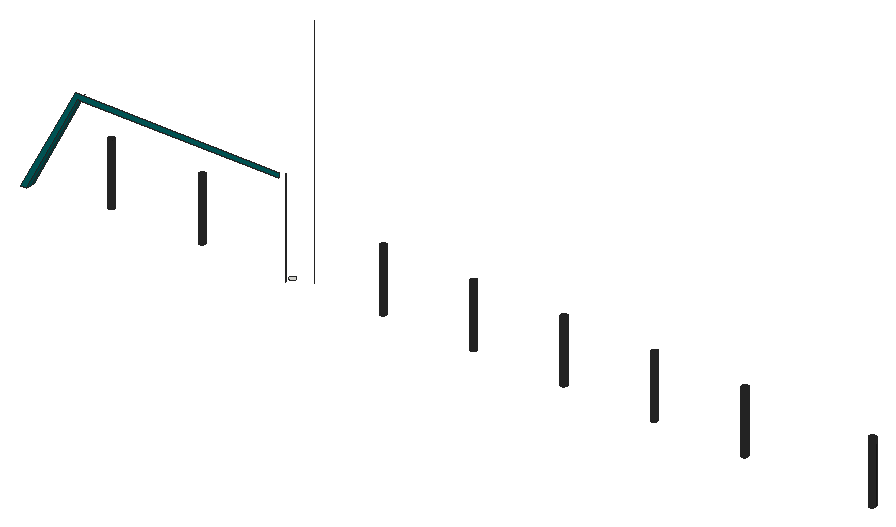
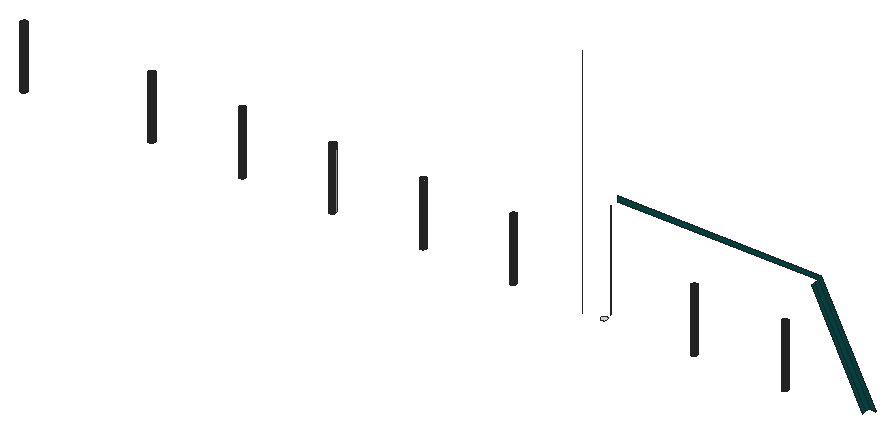
# SketchUp Ruby script. Lengths in inches.
U = 1.inch
M = Sketchup.active_model
def pt(a) = Geom::Point3d.new(a.map { |v| v * U })
def face(e, loops, mat)
  f = e.add_face(loops[0].map { |a| pt(a) })
  loops[1..].each { |l| e.add_face(l.map { |a| pt(a) }).erase! }
  f.material = f.back_material = mat if mat
  f
end
# faces: each face lists its corners as indices into pts; further lists are holes
def faces(e, pts, list, mat = nil) = list.each { |f| face(e, (f[0].is_a?(Array) ? f : [f]).map { |l| l.map { |i| pts[i] } }, mat) }
# xy, xz, yz: faces in a plane at the given z, y or x. An outline is a flat list of corners, or four numbers for a rectangle; further outlines are holes
def ring(l) = l.size == 4 ? [[l[0], l[1]], [l[2], l[1]], [l[2], l[3]], [l[0], l[3]]] : l.each_slice(2).to_a
def flat(e, list, mat, &to3) = list.each { |f| face(e, (f[0].is_a?(Array) ? f : [f]).map { |l| ring(l).map { |u, v| to3.(u, v) } }, mat) }
def xy(e, z, list, mat = nil) = flat(e, list, mat) { |x, y| [x, y, z] }
def xz(e, y, list, mat = nil) = flat(e, list, mat) { |x, z| [x, y, z] }
def yz(e, x, list, mat = nil) = flat(e, list, mat) { |y, z| [x, y, z] }
def lines(e, pts, list) = list.each { |a, b| e.add_line(pt(pts[a]), pt(pts[b])) }
# prism: a flat outline (further loops are holes) pulled along v
def prism(e, loops, v, mat = nil)
  f = face(e, loops, mat); d = Geom::Vector3d.new(v.map { |x| x * U })
  f.pushpull(f.normal.samedirection?(d) ? d.length : -d.length)
end
def box(e, o, s, mat = nil) = prism(e, [[o, [o[0] + s[0], o[1], o[2]], [o[0] + s[0], o[1] + s[1], o[2]], [o[0], o[1] + s[1], o[2]]]], [0, 0, s[2]], mat)
def at(x, y, z, deg = 0) = Geom::Transformation.translation(pt([x, y, z])) * Geom::Transformation.rotation(ORIGIN, Z_AXIS, deg.degrees)
def axes(o, x, y, z) = Geom::Transformation.new([*x, 0, *y, 0, *z, 0, *pt(o).to_a, 1])
def part(name) = M.definitions.add(name)
# library, detail: a bought-in or finely detailed component or shape, given as its bounding box
def library(name, o, s) = part(name).tap { |d| box(d.entities, o, s) }
def detail(e, o, s) = box(e.add_group.entities, o, s)
def put(e, d, t, mat = nil) = e.add_instance(d, t).tap { |i| i.material = mat if mat }
def group(e, t, mat = nil) = e.add_group.tap { |g| g.transformation = t; g.material = mat if mat }.entities
root = M.entities
M.materials.add("[0136_Charcoal]").color = [35, 35, 35]
M.materials.add("[Color H08]").color = [0, 102, 102]
xy(root,420,[[477.27,39.3,476.78,39.36,476.33,39.55,475.94,39.85,475.64,40.24,475.46,40.6875,475.39,41.17,475.46,41.66,475.64,42.11,475.94,42.5,476.33,42.8,476.78,42.98,477.27,43.05,477.75,42.98,478.2,42.8,478.59,42.5,478.89,42.11,479.08,41.66,479.14,41.17,479.08,40.6875,478.89,40.24,478.59,39.85,478.2,39.55,477.75,39.36],[536.27,39.3,535.78,39.36,535.33,39.55,534.94,39.85,534.64,40.24,534.46,40.6875,534.39,41.17,534.46,41.66,534.64,42.11,534.94,42.5,535.33,42.8,535.78,42.98,536.27,43.05,536.75,42.98,537.2,42.8,537.59,42.5,537.89,42.11,538.08,41.66,538.14,41.17,538.08,40.6875,537.89,40.24,537.59,39.85,537.2,39.55,536.75,39.36],[595.27,39.3,594.78,39.36,594.33,39.55,593.94,39.85,593.64,40.24,593.46,40.6875,593.39,41.17,593.46,41.66,593.64,42.11,593.94,42.5,594.33,42.8,594.78,42.98,595.27,43.05,595.75,42.98,596.2,42.8,596.59,42.5,596.89,42.11,597.08,41.66,597.14,41.17,597.08,40.6875,596.89,40.24,596.59,39.85,596.2,39.55,595.75,39.36],[654.27,39.3,653.78,39.36,653.33,39.55,652.94,39.85,652.64,40.24,652.46,40.6875,652.39,41.17,652.46,41.66,652.64,42.11,652.94,42.5,653.33,42.8,653.78,42.98,654.27,43.05,654.75,42.98,655.2,42.8,655.59,42.5,655.89,42.11,656.08,41.66,656.14,41.17,656.08,40.6875,655.89,40.24,655.59,39.85,655.2,39.55,654.75,39.36],[713.27,39.3,712.78,39.36,712.33,39.55,711.94,39.85,711.64,40.24,711.46,40.6875,711.39,41.17,711.46,41.66,711.64,42.11,711.94,42.5,712.33,42.8,712.78,42.98,713.27,43.05,713.75,42.98,714.2,42.8,714.59,42.5,714.89,42.11,715.08,41.66,715.14,41.17,715.08,40.6875,714.89,40.24,714.59,39.85,714.2,39.55,713.75,39.36],
  [772.27,39.3,771.78,39.36,771.33,39.55,770.94,39.85,770.64,40.24,770.46,40.6875,770.39,41.17,770.46,41.66,770.64,42.11,770.94,42.5,771.33,42.8,771.78,42.98,772.27,43.05,772.75,42.98,773.2,42.8,773.59,42.5,773.89,42.11,774.08,41.66,774.14,41.17,774.08,40.6875,773.89,40.24,773.59,39.85,773.2,39.55,772.75,39.36],[831.27,39.3,830.78,39.36,830.33,39.55,829.94,39.85,829.64,40.24,829.46,40.6875,829.39,41.17,829.46,41.66,829.64,42.11,829.94,42.5,830.33,42.8,830.78,42.98,831.27,43.05,831.75,42.98,832.2,42.8,832.59,42.5,832.89,42.11,833.08,41.66,833.14,41.17,833.08,40.6875,832.89,40.24,832.59,39.85,832.2,39.55,831.75,39.36],[890.27,39.3,889.78,39.36,889.33,39.55,888.94,39.85,888.64,40.24,888.46,40.6875,888.39,41.17,888.46,41.66,888.64,42.11,888.94,42.5,889.33,42.8,889.78,42.98,890.27,43.05,890.75,42.98,891.2,42.8,891.59,42.5,891.89,42.11,892.08,41.66,892.14,41.17,892.08,40.6875,891.89,40.24,891.59,39.85,891.2,39.55,890.75,39.36],[973.58,39.3,973.09,39.36,972.64,39.55,972.25,39.85,971.96,40.24,971.77,40.6875,971.7,41.17,971.77,41.66,971.96,42.11,972.25,42.5,972.64,42.8,973.09,42.98,973.58,43.05,974.06,42.98,974.52,42.8,974.91,42.5,975.2,42.11,975.39,41.66,975.45,41.17,975.39,40.6875,975.2,40.24,974.91,39.85,974.52,39.55,974.06,39.36]])
xz(root,30,[[426.66,420,430.89,420,464.4,483.48,595.0625,483.48,595.0625,486.6875,463.18,486.6875]],"[Color H08]")
yz(root,595.0625,[[35.8125,420,36,483.48],[35.8125,420,36,483.48]])
p = [[430.89,33,420],[464.4,33,483.48],[464.4,30,483.48],[430.89,30,420],[464.4,35.8125,483.48],[430.89,35.8125,420],
  [476.78,39.36,420],[477.27,39.3,420],[477.27,39.3,460.3125],[476.78,39.36,460.3125],[477.75,39.36,420],[477.75,39.36,460.3125],
  [535.78,39.36,420],[536.27,39.3,420],[536.27,39.3,460.3125],[535.78,39.36,460.3125],[536.75,39.36,420],[536.75,39.36,460.3125],
  [653.78,39.36,420],[654.27,39.3,420],[654.27,39.3,460.3125],[653.78,39.36,460.3125],[654.75,39.36,420],[654.75,39.36,460.3125],
  [712.78,39.36,420],[713.27,39.3,420],[713.27,39.3,460.3125],[712.78,39.36,460.3125],[713.75,39.36,420],[713.75,39.36,460.3125],
  [771.78,39.36,420],[772.27,39.3,420],[772.27,39.3,460.3125],[771.78,39.36,460.3125],[772.75,39.36,420],[772.75,39.36,460.3125],
  [830.78,39.36,420],[831.27,39.3,420],[831.27,39.3,460.3125],[830.78,39.36,460.3125],[831.75,39.36,420],[831.75,39.36,460.3125],
  [889.78,39.36,420],[890.27,39.3,420],[890.27,39.3,460.3125],[889.78,39.36,460.3125],[890.75,39.36,420],[890.75,39.36,460.3125],
  [973.09,39.36,420],[973.58,39.3,420],[973.58,39.3,460.3125],[973.09,39.36,460.3125],[974.06,39.36,420],[974.06,39.36,460.3125],
  [476.33,39.55,420],[476.33,39.55,460.3125],[478.2,39.55,420],[478.2,39.55,460.3125],[535.33,39.55,420],[535.33,39.55,460.3125],
  [537.2,39.55,420],[537.2,39.55,460.3125],[653.33,39.55,420],[653.33,39.55,460.3125],[655.2,39.55,420],[655.2,39.55,460.3125],
  [712.33,39.55,420],[712.33,39.55,460.3125],[714.2,39.55,420],[714.2,39.55,460.3125],[771.33,39.55,420],[771.33,39.55,460.3125],
  [773.2,39.55,420],[773.2,39.55,460.3125],[830.33,39.55,420],[830.33,39.55,460.3125],[832.2,39.55,420],[832.2,39.55,460.3125],
  [889.33,39.55,420],[889.33,39.55,460.3125],[891.2,39.55,420],[891.2,39.55,460.3125],[972.64,39.55,420],[972.64,39.55,460.3125],
  [974.52,39.55,420],[974.52,39.55,460.3125],[475.94,39.85,420],[475.94,39.85,460.3125],[478.59,39.85,420],[478.59,39.85,460.3125],
  [534.94,39.85,420],[534.94,39.85,460.3125],[537.59,39.85,420],[537.59,39.85,460.3125],[652.94,39.85,420],[652.94,39.85,460.3125],
  [655.59,39.85,420],[655.59,39.85,460.3125],[711.94,39.85,420],[711.94,39.85,460.3125],[714.59,39.85,420],[714.59,39.85,460.3125],
  [770.94,39.85,420],[770.94,39.85,460.3125],[773.59,39.85,420],[773.59,39.85,460.3125],[829.94,39.85,420],[829.94,39.85,460.3125],
  [832.59,39.85,420],[832.59,39.85,460.3125],[888.94,39.85,420],[888.94,39.85,460.3125],[891.59,39.85,420],[891.59,39.85,460.3125],
  [972.25,39.85,420],[972.25,39.85,460.3125],[974.91,39.85,420],[974.91,39.85,460.3125],[475.64,40.24,420],[475.64,40.24,460.3125],
  [478.89,40.24,420],[478.89,40.24,460.3125],[534.64,40.24,420],[534.64,40.24,460.3125],[537.89,40.24,420],[537.89,40.24,460.3125],
  [652.64,40.24,420],[652.64,40.24,460.3125],[655.89,40.24,420],[655.89,40.24,460.3125],[711.64,40.24,420],[711.64,40.24,460.3125],
  [714.89,40.24,420],[714.89,40.24,460.3125],[770.64,40.24,420],[770.64,40.24,460.3125],[773.89,40.24,420],[773.89,40.24,460.3125],
  [829.64,40.24,420],[829.64,40.24,460.3125],[832.89,40.24,420],[832.89,40.24,460.3125],[888.64,40.24,420],[888.64,40.24,460.3125],
  [891.89,40.24,420],[891.89,40.24,460.3125],[971.96,40.24,420],[971.96,40.24,460.3125],[975.2,40.24,420],[975.2,40.24,460.3125],
  [475.46,40.6875,420],[475.46,40.6875,460.3125],[479.08,40.6875,420],[479.08,40.6875,460.3125],[534.46,40.6875,420],[534.46,40.6875,460.3125],
  [538.08,40.6875,420],[538.08,40.6875,460.3125],[652.46,40.6875,420],[652.46,40.6875,460.3125],[656.08,40.6875,420],[656.08,40.6875,460.3125],
  [711.46,40.6875,420],[711.46,40.6875,460.3125],[715.08,40.6875,420],[715.08,40.6875,460.3125],[770.46,40.6875,420],[770.46,40.6875,460.3125],
  [774.08,40.6875,420],[774.08,40.6875,460.3125],[829.46,40.6875,420],[829.46,40.6875,460.3125],[833.08,40.6875,420],[833.08,40.6875,460.3125],
  [888.46,40.6875,420],[888.46,40.6875,460.3125],[892.08,40.6875,420],[892.08,40.6875,460.3125],[971.77,40.6875,420],[971.77,40.6875,460.3125],
  [975.39,40.6875,420],[975.39,40.6875,460.3125],[475.39,41.17,420],[475.39,41.17,460.3125],[479.14,41.17,420],[479.14,41.17,460.3125],
  [534.39,41.17,420],[534.39,41.17,460.3125],[538.14,41.17,420],[538.14,41.17,460.3125],[652.39,41.17,420],[652.39,41.17,460.3125],
  [656.14,41.17,420],[656.14,41.17,460.3125],[711.39,41.17,420],[711.39,41.17,460.3125],[715.14,41.17,420],[715.14,41.17,460.3125],
  [770.39,41.17,420],[770.39,41.17,460.3125],[774.14,41.17,420],[774.14,41.17,460.3125],[829.39,41.17,420],[829.39,41.17,460.3125],
  [833.14,41.17,420],[833.14,41.17,460.3125],[888.39,41.17,420],[888.39,41.17,460.3125],[892.14,41.17,420],[892.14,41.17,460.3125],
  [971.7,41.17,420],[971.7,41.17,460.3125],[975.45,41.17,420],[975.45,41.17,460.3125],[475.46,41.66,420],[475.46,41.66,460.3125],
  [479.08,41.66,420],[479.08,41.66,460.3125],[534.46,41.66,420],[534.46,41.66,460.3125],[538.08,41.66,420],[538.08,41.66,460.3125],
  [652.46,41.66,420],[652.46,41.66,460.3125],[656.08,41.66,420],[656.08,41.66,460.3125],[711.46,41.66,420],[711.46,41.66,460.3125],
  [715.08,41.66,420],[715.08,41.66,460.3125],[770.46,41.66,420],[770.46,41.66,460.3125],[774.08,41.66,420],[774.08,41.66,460.3125],
  [829.46,41.66,420],[829.46,41.66,460.3125],[833.08,41.66,420],[833.08,41.66,460.3125],[888.46,41.66,420],[888.46,41.66,460.3125],
  [892.08,41.66,420],[892.08,41.66,460.3125],[971.77,41.66,420],[971.77,41.66,460.3125],[975.39,41.66,420],[975.39,41.66,460.3125],
  [475.64,42.11,420],[475.64,42.11,460.3125],[478.89,42.11,420],[478.89,42.11,460.3125],[534.64,42.11,420],[534.64,42.11,460.3125],
  [537.89,42.11,420],[537.89,42.11,460.3125],[652.64,42.11,420],[652.64,42.11,460.3125],[655.89,42.11,420],[655.89,42.11,460.3125],
  [711.64,42.11,420],[711.64,42.11,460.3125],[714.89,42.11,420],[714.89,42.11,460.3125],[770.64,42.11,420],[770.64,42.11,460.3125],
  [773.89,42.11,420],[773.89,42.11,460.3125],[829.64,42.11,420],[829.64,42.11,460.3125],[832.89,42.11,420],[832.89,42.11,460.3125],
  [888.64,42.11,420],[888.64,42.11,460.3125],[891.89,42.11,420],[891.89,42.11,460.3125],[971.96,42.11,420],[971.96,42.11,460.3125],
  [975.2,42.11,420],[975.2,42.11,460.3125],[475.94,42.5,420],[475.94,42.5,460.3125],[478.59,42.5,420],[478.59,42.5,460.3125],
  [534.94,42.5,420],[534.94,42.5,460.3125],[537.59,42.5,420],[537.59,42.5,460.3125],[652.94,42.5,420],[652.94,42.5,460.3125],
  [655.59,42.5,420],[655.59,42.5,460.3125],[711.94,42.5,420],[711.94,42.5,460.3125],[714.59,42.5,420],[714.59,42.5,460.3125],
  [770.94,42.5,420],[770.94,42.5,460.3125],[773.59,42.5,420],[773.59,42.5,460.3125],[829.94,42.5,420],[829.94,42.5,460.3125],
  [832.59,42.5,420],[832.59,42.5,460.3125],[888.94,42.5,420],[888.94,42.5,460.3125],[891.59,42.5,420],[891.59,42.5,460.3125],
  [972.25,42.5,420],[972.25,42.5,460.3125],[974.91,42.5,420],[974.91,42.5,460.3125],[476.33,42.8,420],[476.33,42.8,460.3125],
  [478.2,42.8,420],[478.2,42.8,460.3125],[535.33,42.8,420],[535.33,42.8,460.3125],[537.2,42.8,420],[537.2,42.8,460.3125],
  [653.33,42.8,420],[653.33,42.8,460.3125],[655.2,42.8,420],[655.2,42.8,460.3125],[712.33,42.8,420],[712.33,42.8,460.3125],
  [714.2,42.8,420],[714.2,42.8,460.3125],[771.33,42.8,420],[771.33,42.8,460.3125],[773.2,42.8,420],[773.2,42.8,460.3125],
  [830.33,42.8,420],[830.33,42.8,460.3125],[832.2,42.8,420],[832.2,42.8,460.3125],[889.33,42.8,420],[889.33,42.8,460.3125],
  [891.2,42.8,420],[891.2,42.8,460.3125],[972.64,42.8,420],[972.64,42.8,460.3125],[974.52,42.8,420],[974.52,42.8,460.3125],
  [476.78,42.98,420],[476.78,42.98,460.3125],[477.75,42.98,420],[477.75,42.98,460.3125],[535.78,42.98,420],[535.78,42.98,460.3125],
  [536.75,42.98,420],[536.75,42.98,460.3125],[653.78,42.98,420],[653.78,42.98,460.3125],[654.75,42.98,420],[654.75,42.98,460.3125],
  [712.78,42.98,420],[712.78,42.98,460.3125],[713.75,42.98,420],[713.75,42.98,460.3125],[771.78,42.98,420],[771.78,42.98,460.3125],
  [772.75,42.98,420],[772.75,42.98,460.3125],[830.78,42.98,420],[830.78,42.98,460.3125],[831.75,42.98,420],[831.75,42.98,460.3125],
  [889.78,42.98,420],[889.78,42.98,460.3125],[890.75,42.98,420],[890.75,42.98,460.3125],[973.09,42.98,420],[973.09,42.98,460.3125],
  [973.09,42.98,458.74],[973.09,42.98,455.81],[974.06,42.98,420],[974.06,42.98,460.3125],[477.27,43.05,420],[477.27,43.05,460.3125],
  [536.27,43.05,420],[536.27,43.05,460.3125],[654.27,43.05,420],[654.27,43.05,460.3125],[713.27,43.05,420],[713.27,43.05,460.3125],
  [772.27,43.05,420],[772.27,43.05,460.3125],[831.27,43.05,420],[831.27,43.05,460.3125],[890.27,43.05,420],[890.27,43.05,460.3125],
  [973.58,43.05,420],[973.58,43.05,460.3125],[973.58,43.05,424.01],[973.58,43.05,421.17],[607.2,44.0625,420],[607.2,44.0625,573.81]]
faces(root,p,[[0,1,2,3],[0,1,4,5]],"[Color H08]")
faces(root,p,[[6,7,8,9],[7,10,11,8],[12,13,14,15],[13,16,17,14],[36,37,38,39],[37,40,41,38],[42,43,44,45],[43,46,47,44],
  [48,49,50,51],[49,52,53,50],[54,6,9,55],[10,56,57,11],[58,12,15,59],[16,60,61,17],[74,36,39,75],[40,76,77,41],
  [78,42,45,79],[46,80,81,47],[82,48,51,83],[52,84,85,53],[86,54,55,87],[56,88,89,57],[90,58,59,91],[60,92,93,61],
  [106,74,75,107],[76,108,109,77],[110,78,79,111],[80,112,113,81],[114,82,83,115],[84,116,117,85],[118,86,87,119],[88,120,121,89],
  [122,90,91,123],[92,124,125,93],[138,106,107,139],[108,140,141,109],[142,110,111,143],[112,144,145,113],[146,114,115,147],[116,148,149,117],
  [150,118,119,151],[120,152,153,121],[154,122,123,155],[124,156,157,125],[170,138,139,171],[140,172,173,141],[174,142,143,175],[144,176,177,145],
  [178,146,147,179],[148,180,181,149],[182,150,151,183],[152,184,185,153],[186,154,155,187],[156,188,189,157],[202,170,171,203],[172,204,205,173],
  [206,174,175,207],[176,208,209,177],[210,178,179,211],[180,212,213,181],[214,182,183,215],[184,216,217,185],[218,186,187,219],[188,220,221,189],
  [234,202,203,235],[204,236,237,205],[238,206,207,239],[208,240,241,209],[242,210,211,243],[212,244,245,213],[246,214,215,247],[216,248,249,217],
  [250,218,219,251],[220,252,253,221],[266,234,235,267],[236,268,269,237],[270,238,239,271],[240,272,273,241],[274,242,243,275],[244,276,277,245],
  [278,246,247,279],[248,280,281,249],[282,250,251,283],[252,284,285,253],[298,266,267,299],[268,300,301,269],[302,270,271,303],[272,304,305,273],
  [306,274,275,307],[276,308,309,277],[310,278,279,311],[280,312,313,281],[314,282,283,315],[284,316,317,285],[330,298,299,331],[300,332,333,301],
  [334,302,303,335],[304,336,337,305],[338,306,307,339],[308,340,341,309],[342,310,311,343],[312,344,345,313],[346,314,315,347],[316,348,349,317],
  [362,330,331,363],[332,364,365,333],[366,334,335,367],[336,368,369,337],[370,338,339,371,372,373],[340,374,375,341],[376,342,343,377],[344,376,377,345],
  [378,346,347,379],[348,378,379,349],[386,362,363,387],[364,386,387,365],[388,366,367,389],[368,388,389,369],[390,370,373,372,371,391,392,393],[374,390,393,392,391,375]],"[0136_Charcoal]")
faces(root,p,[[18,19,20,21],[19,22,23,20],[24,25,26,27],[25,28,29,26],[30,31,32,33],[31,34,35,32],[62,18,21,63],[22,64,65,23],
  [66,24,27,67],[28,68,69,29],[70,30,33,71],[34,72,73,35],[94,62,63,95],[64,96,97,65],[98,66,67,99],[68,100,101,69],
  [102,70,71,103],[72,104,105,73],[126,94,95,127],[96,128,129,97],[130,98,99,131],[100,132,133,101],[134,102,103,135],[104,136,137,105],
  [158,126,127,159],[128,160,161,129],[162,130,131,163],[132,164,165,133],[166,134,135,167],[136,168,169,137],[190,158,159,191],[160,192,193,161],
  [194,162,163,195],[164,196,197,165],[198,166,167,199],[168,200,201,169],[222,190,191,223],[192,224,225,193],[226,194,195,227],[196,228,229,197],
  [230,198,199,231],[200,232,233,201],[254,222,223,255],[224,256,257,225],[258,226,227,259],[228,260,261,229],[262,230,231,263],[232,264,265,233],
  [286,254,255,287],[256,288,289,257],[290,258,259,291],[260,292,293,261],[294,262,263,295],[264,296,297,265],[318,286,287,319],[288,320,321,289],
  [322,290,291,323],[292,324,325,293],[326,294,295,327],[296,328,329,297],[350,318,319,351],[320,352,353,321],[354,322,323,355],[324,356,357,325],
  [358,326,327,359],[328,360,361,329],[380,350,351,381],[352,380,381,353],[382,354,355,383],[356,382,383,357],[384,358,359,385],[360,384,385,361]])
lines(root,p,[[394,395]])
